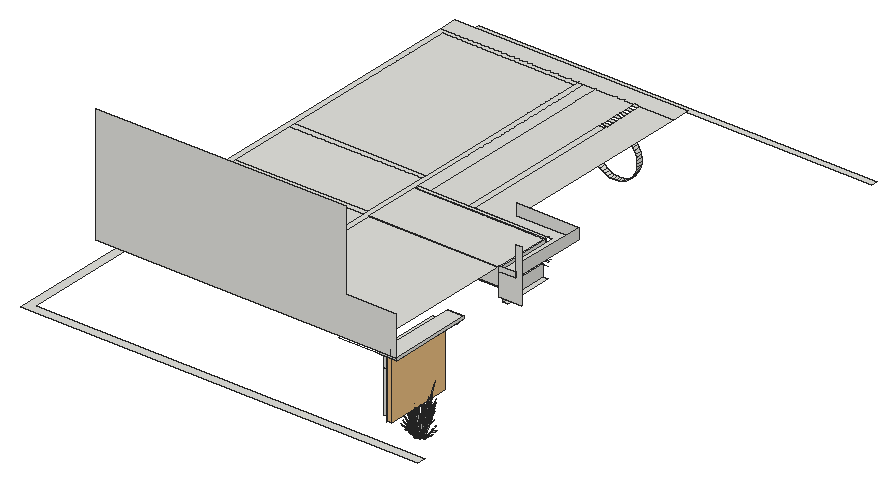
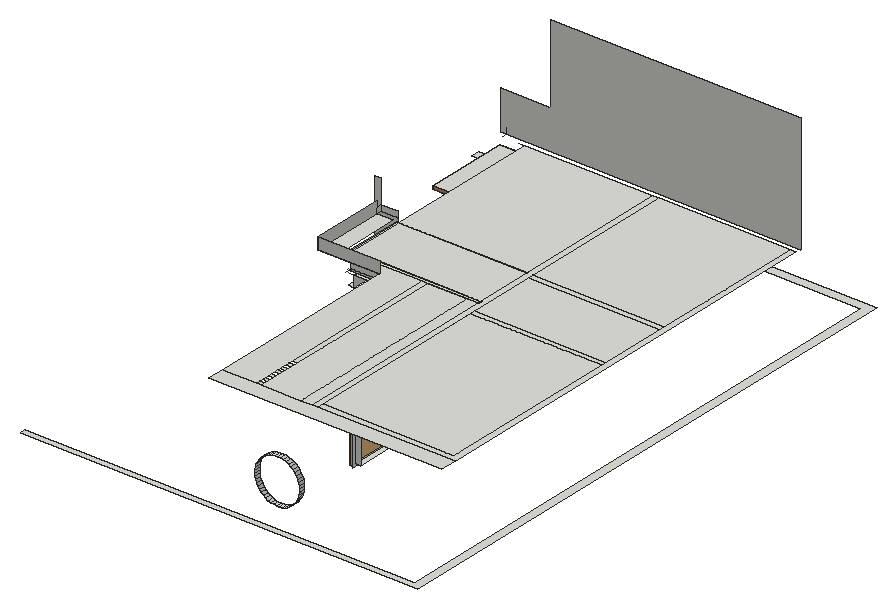
# SketchUp Ruby script. Lengths in inches.
U = 1.inch
M = Sketchup.active_model
def pt(a) = Geom::Point3d.new(a.map { |v| v * U })
def face(e, loops, mat)
  f = e.add_face(loops[0].map { |a| pt(a) })
  loops[1..].each { |l| e.add_face(l.map { |a| pt(a) }).erase! }
  f.material = f.back_material = mat if mat
  f
end
# faces: each face lists its corners as indices into pts; further lists are holes
def faces(e, pts, list, mat = nil) = list.each { |f| face(e, (f[0].is_a?(Array) ? f : [f]).map { |l| l.map { |i| pts[i] } }, mat) }
# xy, xz, yz: faces in a plane at the given z, y or x. An outline is a flat list of corners, or four numbers for a rectangle; further outlines are holes
def ring(l) = l.size == 4 ? [[l[0], l[1]], [l[2], l[1]], [l[2], l[3]], [l[0], l[3]]] : l.each_slice(2).to_a
def flat(e, list, mat, &to3) = list.each { |f| face(e, (f[0].is_a?(Array) ? f : [f]).map { |l| ring(l).map { |u, v| to3.(u, v) } }, mat) }
def xy(e, z, list, mat = nil) = flat(e, list, mat) { |x, y| [x, y, z] }
def xz(e, y, list, mat = nil) = flat(e, list, mat) { |x, z| [x, y, z] }
def yz(e, x, list, mat = nil) = flat(e, list, mat) { |y, z| [x, y, z] }
def lines(e, pts, list) = list.each { |a, b| e.add_line(pt(pts[a]), pt(pts[b])) }
# prism: a flat outline (further loops are holes) pulled along v
def prism(e, loops, v, mat = nil)
  f = face(e, loops, mat); d = Geom::Vector3d.new(v.map { |x| x * U })
  f.pushpull(f.normal.samedirection?(d) ? d.length : -d.length)
end
def box(e, o, s, mat = nil) = prism(e, [[o, [o[0] + s[0], o[1], o[2]], [o[0] + s[0], o[1] + s[1], o[2]], [o[0], o[1] + s[1], o[2]]]], [0, 0, s[2]], mat)
def at(x, y, z, deg = 0) = Geom::Transformation.translation(pt([x, y, z])) * Geom::Transformation.rotation(ORIGIN, Z_AXIS, deg.degrees)
def axes(o, x, y, z) = Geom::Transformation.new([*x, 0, *y, 0, *z, 0, *pt(o).to_a, 1])
def part(name) = M.definitions.add(name)
# library, detail: a bought-in or finely detailed component or shape, given as its bounding box
def library(name, o, s) = part(name).tap { |d| box(d.entities, o, s) }
def detail(e, o, s) = box(e.add_group.entities, o, s)
def put(e, d, t, mat = nil) = e.add_instance(d, t).tap { |i| i.material = mat if mat }
def group(e, t, mat = nil) = e.add_group.tap { |g| g.transformation = t; g.material = mat if mat }.entities
root = M.entities
M.materials.add("Brick_10_1K").color = [200, 136, 115]
M.materials.add("LightPink_Translucent").color = [144, 107, 117]
M.materials["LightPink_Translucent"].alpha = 0.75
c1 = part("blade")
p = [[2.15,0.21,22],[0,0.17,0],[0.09,0.45,0],[2.18,0.31,22],[2.29,0.31,22],[0.38,0.45,0],
  [2.48,0.24,33],[2.49,0.24,33],[2.48,0.22,33]]
faces(c1.entities,p,[[0,1,2,3],[4,5,2,3],[6,3,4,7],[8,0,3,6]])
c2 = part("seeds")
p = [[0.3,-0.1,1.38],[-0.01,-0.03,1.59],[-0.01,-0.03,0.03],[0.14,-0.07,-0.07],[0.29,-0.03,3],[0.15,0.01,3.11]]
faces(c2.entities,p,[[0,1,2,3],[1,0,4,5]],"LightPink_Translucent")
c3 = part("blade with seeds")
put(c3.entities,c1,at(0,0,0))
put(c3.entities,c2,axes([2.4,0.25,30.99],[1.5799,-0.05474,1.17369],[-0.12525,1.92788,0.29478],[-0.07173,-0.02425,1.56792]))
c4 = library("mesh-162",[-1607.75,-1245.64,-53.98],[1739.16,1702.88,120.91])
c5 = part("Group9\#1")
put(c5.entities,c4,at(0,0,0))
xy(root,39,[[192,384,198,450]])
xy(root,45,[[336,66,342,111],[336,111,342,132]])
xy(root,60,[[0,0,426,0,426,9,9,9,9,606.89,426,606.89,426,612.89,0,612.89]])
xy(root,84,[[336,225,342,279]])
xy(root,93,[[192,324,198,366],[192,384,198,450]])
xy(root,96,[[198,225,336,279]])
xy(root,111,[[342,54,360,63],[342,63,360,66],[336,66,360,132],[342,132,360,135],[342,135,360,138.72]])
xy(root,111,[[342,138.72,360,144]],"Brick_10_1K")
xy(root,114,[[342,54,360,144]])
xy(root,120,[[45,51,51,51,51,501,192,501,192,507,45,507],[51,51,192,219],[192,51,198,507],[198,51,336,219],[51,219,192,225],
  [198,219,336,281],[342,219,342,285,258,285,258,507,294,507,294,297,360,297,360,219],[336,219,338,281],[51,225,192,297],[198,281,336,285],
  [336,281,338,285],[198,285,210,507],[210,285,252,507],[252,285,258,459],[51,297,192,303],
  [51,303,192,501],[252,463,258,467],[252,471,258,475],[252,479,258,483],[252,487,258,491],
  [252,495,258,499],[252,503,258,507],[45,507,294,525]])
xz(root,45,[[45,120,366,120,366,162,312,162,312,246,45,246]])
xz(root,54,[[342,111,360,114]])
xz(root,66,[[336,45,342,90],[336,90,342,111]])
xz(root,132,[[336,45,342,111]])
xz(root,144,[[342,111,360,114]],"Brick_10_1K")
xz(root,213,[[342,96,366,96,366,151.99,360,151.99,360,120,342,120],[342,120,360,126]])
xz(root,219,[[198,102,336,120],[336,102,338,120]])
xz(root,281,[[198,100,338,102],[198,102,338,120]])
xz(root,297,[[294,120,360,132]])
xz(root,384,[[192,39,198,93]])
xz(root,450,[[192,39,198,93]])
yz(root,198,[[[381,36,453,96],[384,39,450,93]],[281,100,285,120]])
yz(root,336,[[225,84,279,96]])
yz(root,338,[[225,100,279,102],[279,100,281,102],[219,102,279,120]])
yz(root,342,[[63,42,135,42,135,111,132,111,132,45,66,45,66,111,63,111]])
yz(root,360,[[54,111,144,114],[213,120,219,126],[219,120,297,132]])
p = [[217.42,531,27.05],[214.41,531,27.11],[214.41,525,27.11],[217.42,525,27.05],[220.42,531,27.36],[220.42,525,27.36],
  [211.43,531,27.55],[211.43,525,27.55],[223.35,531,28.05],[223.35,525,28.05],[208.52,531,28.36],[208.52,525,28.36],
  [226.18,531,29.1],[226.18,525,29.1],[205.74,531,29.53],[205.74,525,29.53],[228.85,531,30.5],[228.85,525,30.5],
  [203.13,531,31.04],[203.13,525,31.04],[231.32,531,32.22],[231.32,525,32.22],[200.73,531,32.86],[200.73,525,32.86],
  [233.5625,531,34.24],[233.5625,525,34.24],[198.58,531,34.97],[198.58,525,34.97],[235.53,531,36.52],[235.53,525,36.52],
  [196.71,531,37.33],[196.71,525,37.33],[237.2,531,39.03],[237.2,525,39.03],[195.15,531,39.91],[195.15,525,39.91],
  [238.54,531,41.73],[238.54,525,41.73],[193.92,531,42.66],[193.92,525,42.66],[239.53,531,44.58],[239.53,525,44.58],
  [193.05,531,45.54],[193.05,525,45.54],[240.16,531,47.52],[240.16,525,47.52],[192.55,531,48.52],[192.55,525,48.52],
  [240.41,531,50.53],[240.41,525,50.53],[192.42,531,51.53],[192.42,525,51.53],[240.28,531,53.54],[240.28,525,53.54],
  [192.67,531,54.53],[192.67,525,54.53],[239.78,531,56.51],[239.78,525,56.51],[193.3,531,57.48],[193.3,525,57.48],
  [238.91,531,59.4],[238.91,525,59.4],[194.29,531,60.33],[194.29,525,60.33],[237.68,531,62.15],[237.68,525,62.15],
  [195.63,531,63.03],[195.63,525,63.03],[236.12,531,64.73],[236.12,525,64.73],[197.3,531,65.54],[197.3,525,65.54],
  [234.25,531,67.09],[234.25,525,67.09],[199.27,531,67.82],[199.27,525,67.82],[232.09,531,69.2],[232.09,525,69.2],
  [201.5,531,69.83],[201.5,525,69.83],[229.69,531,71.02],[229.69,525,71.02],[203.98,531,71.55],[203.98,525,71.55],
  [227.08,531,72.53],[227.08,525,72.53],[206.65,531,72.95],[206.65,525,72.95],[224.3,531,73.69],[224.3,525,73.69],
  [209.48,531,74],[209.48,525,74],[221.4,531,74.5],[221.4,525,74.5],[212.41,531,74.69],[212.41,525,74.69],
  [218.42,531,74.94],[218.42,525,74.94],[215.41,531,75.01],[215.41,525,75.01],[340,283,100],[340,285,100],
  [342,54,111],[297.24,54,111],[338,281,100],[342,281,100],[338,225,100],[342,225,100],
  [338,279,100],[342,279,100],[336,225,96],[342,225,96],[336,279,96],[342,279,96],
  [360,45,120],[360,45,126],[360,51,120],[336,51,120],[342,51,120]]
faces(root,p,[[0,1,2,3],[4,0,3,5],[1,6,7,2],[8,4,5,9],[6,10,11,7],[12,8,9,13],[10,14,15,11],[16,12,13,17],
  [14,18,19,15],[20,16,17,21],[18,22,23,19],[24,20,21,25],[22,26,27,23],[28,24,25,29],[26,30,31,27],[32,28,29,33],
  [30,34,35,31],[36,32,33,37],[34,38,39,35],[40,36,37,41],[38,42,43,39],[44,40,41,45],[42,46,47,43],[48,44,45,49],
  [46,50,51,47],[52,48,49,53],[50,54,55,51],[56,52,53,57],[54,58,59,55],[60,56,57,61],[58,62,63,59],[64,60,61,65],
  [62,66,67,63],[68,64,65,69],[66,70,71,67],[72,68,69,73],[70,74,75,71],[76,72,73,77],[74,78,79,75],[80,76,77,81],
  [78,82,83,79],[84,80,81,85],[82,86,87,83],[88,84,85,89],[86,90,91,87],[92,88,89,93],[90,94,95,91],[96,92,93,97],
  [94,98,99,95],[98,96,97,99]])
lines(root,p,[[100,101],[102,103],[104,105],[106,107],[108,109],[110,111],[112,113],[114,115],[116,114],[117,118]])
put(root,c3,axes([347.28,106.03,11.03],[0.0479,-0.66354,-0.1216],[0.90696,0.01814,-0.67495],[0.3493,0.04609,1.02557]))
put(root,c3,axes([340.5,103.49,11.03],[0.45012,0.59081,-0.1216],[-0.79888,0.29033,-0.67495],[-0.33665,0.07795,1.02557]))
put(root,c3,axes([347.19,102.2,11.03],[-0.98321,-0.03233,-0.1216],[0.02687,-0.61208,-0.67495],[0.0683,-0.23574,1.02557]))
put(root,c3,axes([348.29,104.8,11.03],[-0.45012,-0.59081,-0.1216],[0.79888,-0.29033,-0.67495],[0.33665,-0.07795,1.02557]))
put(root,c3,axes([343.42,106.78,11.03],[0.87543,-0.30377,-0.1216],[0.4302,0.53915,-0.67495],[0.1155,0.2272,1.02557]))
put(root,c3,axes([341.51,102.26,11.03],[-0.0479,0.66354,-0.1216],[-0.90696,-0.01814,-0.67495],[-0.3493,-0.04609,1.02557]))
put(root,c3,axes([345.5,106.75,11.03],[0.53309,-0.55848,-0.1216],[0.77201,0.32175,-0.67495],[0.26836,0.15779,1.02557]))
put(root,c3,axes([340.53,104.89,11.03],[0.82753,0.35977,-0.1216],[-0.47675,0.52101,-0.67495],[-0.2338,0.18111,1.02557]))
put(root,c3,axes([345.37,101.51,11.03],[-0.87543,0.30377,-0.1216],[-0.4302,-0.53915,-0.67495],[-0.1155,-0.2272,1.02557]))
put(root,c3,axes([348.26,103.4,11.03],[-0.82753,-0.35977,-0.1216],[0.47675,-0.52101,-0.67495],[0.2338,-0.18111,1.02557]))
put(root,c3,axes([346.1,103.46,10.47],[-0.77304,-0.33901,1.38283],[0.81626,-0.52782,0.59665],[0.24941,0.31809,1.33663]))
put(root,c3,axes([339.56,104.08,10.72],[-0.14609,0.08471,1.74944],[0.01243,0.61893,-0.27667],[-0.33486,0.08049,0.14031]))
put(root,c3,axes([350.74,103.88,10.72],[0.12414,-0.09938,1.74944],[-0.15889,-0.60963,-0.27667],[0.31148,-0.11559,0.14031]))
put(root,c3,axes([348.07,105.63,10.72],[0.19191,-0.01103,1.74944],[0.52639,-0.5069,-0.27667],[0.34136,0.06691,0.14031]))
put(root,c3,axes([348.09,101.22,10.72],[-0.00864,-0.12985,1.74944],[-0.72937,-0.3753,-0.27667],[0.11277,-0.2275,0.14031]))
put(root,c3,axes([339.58,106.39,10.72],[-0.02224,0.12912,1.74944],[0.63107,0.44917,-0.27667],[-0.16521,0.21241,0.14031]))
put(root,c3,axes([343.21,107.98,10.72],[0.1134,0.10507,1.74944],[0.91515,0.04128,-0.27667],[0.09203,0.23172,0.14031]))
put(root,c3,axes([343.98,100.1,10.72],[-0.13683,-0.09148,1.74944],[-0.91315,0.058,-0.27667],[-0.14574,-0.2188,0.14031]))
put(root,c3,axes([340.99,101.11,10.72],[-0.19249,-0.00461,1.74944],[-0.61281,0.46055,-0.27667],[-0.32697,-0.0941,0.14031]))
put(root,c3,axes([340.25,101.5,10.71],[0.06632,0.06511,1.77383],[-0.31973,0.58531,-0.16761],[-0.32381,0.00424,0.31391]))
put(root,c3,axes([343.05,99.8,10.71],[-0.01669,0.07821,1.77383],[-0.82314,0.28383,-0.16761],[-0.24223,-0.14508,0.31391]))
put(root,c3,axes([344.8,107.22,10.71],[0.00265,-0.07899,1.77383],[0.76665,-0.34851,-0.16761],[0.2663,0.12439,0.31391]))
put(root,c3,axes([337.93,104.7,10.71],[0.11417,0.0175,1.77383],[0.35319,0.57649,-0.16761],[-0.23371,0.15131,0.31391]))
put(root,c3,axes([350.3,103.24,10.71],[-0.11685,-0.00496,1.77383],[-0.48522,-0.53096,-0.16761],[0.19486,-0.17458,0.31391]))
put(root,c3,axes([350.09,106.56,10.71],[-0.08089,-0.05712,1.77383],[0.17695,-0.61228,-0.16761],[0.31864,-0.03912,0.31391]))
put(root,c3,axes([339.51,107.71,10.71],[0.10149,-0.03939,1.77383],[0.83886,0.26202,-0.16761],[-0.01971,0.21816,0.31391]))
put(root,c3,axes([347.89,100.76,10.71],[-0.09085,0.04984,1.77383],[-0.89014,-0.16814,-0.16761],[-0.03222,-0.21748,0.31391]))
put(root,c3,axes([341.6,106.09,11.4],[0.98321,0.03233,-0.13498],[-0.02687,0.61208,-0.74919],[-0.0683,0.23574,1.13838]))
put(root,c3,axes([343.28,101.29,11.43],[-0.59706,0.6255,-0.13619],[-0.86465,-0.36036,-0.75594],[-0.30056,-0.17672,1.14864]))
put(root,c3,axes([343.09,101.33,10.73],[0.4066,-0.41448,0.0643],[0.57901,0.24131,0.50621],[-0.18719,-0.13288,0.77189]))
put(root,c3,axes([343.4375,107.02,10.73],[-0.6592,0.22175,0.0643],[-0.32265,-0.40436,0.50621],[0.06366,0.17825,0.77189]))
put(root,c3,axes([348.5625,103.27,10.73],[0.61415,0.2744,0.0643],[-0.35756,0.39076,0.50621],[0.1969,-0.12633,0.77189]))
put(root,c3,axes([348.66,104.79,10.73],[0.32857,0.44488,0.0643],[-0.59916,0.21775,0.50621],[0.26412,-0.04296,0.77189]))
put(root,c3,axes([341.19,102.15,10.73],[0.04505,-0.49615,0.0643],[0.68022,0.0136,0.50621],[-0.26056,-0.05192,0.77189]))
put(root,c3,axes([347.36,101.98,10.73],[0.73517,0.0304,0.0643],[-0.02016,0.45906,0.50621],[0.07693,-0.17585,0.77189]))
put(root,c3,axes([347.61,106.14,10.73],[-0.04505,0.49615,0.0643],[-0.68022,-0.0136,0.50621],[0.26056,0.05192,0.77189]))
put(root,c3,axes([340.23,105.02,10.73],[-0.61415,-0.2744,0.0643],[0.35756,-0.39076,0.50621],[-0.1969,0.12633,0.77189]))
put(root,c3,axes([345.35,101.27,10.73],[0.6592,-0.22175,0.0643],[0.32265,0.40436,0.50621],[-0.06366,-0.17825,0.77189]))
put(root,c3,axes([340.14,103.5,10.73],[-0.32857,-0.44488,0.0643],[0.59916,-0.21775,0.50621],[-0.26412,0.04296,0.77189]))
put(root,c3,axes([345.7,106.96,10.73],[-0.4066,0.41448,0.0643],[-0.57901,-0.24131,0.50621],[0.18719,0.13288,0.77189]))
put(root,c3,axes([341.4375,106.3125,10.73],[-0.73517,-0.0304,0.0643],[0.02016,-0.45906,0.50621],[-0.07693,0.17585,0.77189]))
put(root,c3,axes([345.12,101.3125,10.73],[0.88151,0.17057,0.48003],[-0.30143,0.56078,0.3958],[-0.05297,-0.22053,0.9933]))
put(root,c3,axes([347.67,105.98,10.73],[-0.65964,0.42992,0.48003],[-0.5689,-0.45657,0.3958],[0.30948,0.0793,0.9933]))
put(root,c3,axes([348.59,104.63,10.73],[-0.25275,0.59491,0.48003],[-0.83094,-0.20343,0.3958],[0.32677,-0.03575,0.9933]))
put(root,c3,axes([340.4,105.14,10.73],[-0.22187,-0.60049,0.48003],[0.87033,-0.10422,0.3958],[-0.25651,0.14123,0.9933]))
put(root,c3,axes([341.67,106.35,10.73],[-0.63704,-0.44518,0.48003],[0.67652,-0.38394,0.3958],[-0.11751,0.20886,0.9933]))
put(root,c3,axes([347.12,101.9375,10.73],[0.63704,0.44518,0.48003],[-0.67652,0.38394,0.3958],[0.11751,-0.20886,0.9933]))
put(root,c3,axes([340.2,103.66,10.73],[0.25275,-0.59491,0.48003],[0.83094,0.20343,0.3958],[-0.32677,0.03575,0.9933]))
put(root,c3,axes([348.39,103.15,10.73],[0.22187,0.60049,0.48003],[-0.87033,0.10422,0.3958],[0.25651,-0.14123,0.9933]))
put(root,c3,axes([345.87,106.84,10.73],[-0.88979,0.14973,0.48003],[-0.15442,-0.58737,0.3958],[0.20926,0.17311,0.9933]))
put(root,c3,axes([343.68,106.57,11.05],[0.2697,-0.50175,0.35414],[0.78684,0.14635,-0.4572],[0.07215,0.20201,0.87481]))
put(root,c3,axes([345.11,101.72,11.05],[-0.2697,0.50175,0.35414],[-0.78684,-0.14635,-0.4572],[-0.07215,-0.20201,0.87481]))
put(root,c3,axes([347.14,105.77,11.05],[-0.50902,-0.40851,0.35414],[0.58122,-0.38671,-0.4572],[0.29531,0.05884,0.87481]))
put(root,c3,axes([347.98,104.625,11.05],[-0.74348,-0.18202,0.35414],[0.21685,-0.53102,-0.4572],[0.29933,-0.04869,0.87481]))
put(root,c3,axes([341.65,102.52,11.05],[0.50902,0.40851,0.35414],[-0.58122,0.38671,-0.4572],[-0.29531,-0.05884,0.87481]))
put(root,c3,axes([341.98,106,11.05],[0.60531,-0.34352,0.35414],[0.573,0.39225,-0.4572],[-0.08718,0.19929,0.87481]))
put(root,c3,axes([340.93,104.9375,11.05],[0.77872,-0.09325,0.35414],[0.20563,0.53305,-0.4572],[-0.22316,0.14318,0.87481]))
put(root,c3,axes([345.57,106.48,11.05],[-0.13817,-0.52554,0.35414],[0.78985,-0.13877,-0.4572],[0.21215,0.1506,0.87481]))
put(root,c3,axes([347.86,103.35,11.05],[-0.77872,0.09325,0.35414],[-0.20563,-0.53305,-0.4572],[0.22316,-0.14318,0.87481]))
put(root,c3,axes([340.81,103.66,11.05],[0.74348,0.18202,0.35414],[-0.21685,0.53102,-0.4572],[-0.29933,0.04869,0.87481]))
put(root,c3,axes([346.81,102.29,11.05],[-0.60531,0.34352,0.35414],[-0.573,-0.39225,-0.4572],[0.08718,-0.19929,0.87481]))
put(root,c3,axes([343.22,101.81,11.05],[0.13817,0.52554,0.35414],[-0.78985,0.13877,-0.4572],[-0.21215,-0.1506,0.87481]))
put(root,c3,axes([343.67,106.98,11.0625],[-0.88151,-0.17057,0.53283],[0.30143,-0.56078,0.43934],[0.05297,0.22053,1.10256]))
put(root,c3,axes([340.85,102.15,11.09],[0.7388,-0.48151,0.53763],[0.63717,0.51135,0.4433],[-0.34662,-0.08882,1.11249]))
put(root,c3,axes([342.87,101.19,11.09],[0.99656,-0.1677,0.53763],[0.17295,0.65785,0.4433],[-0.23438,-0.19388,1.11249]))
put(root,c3,axes([344.74,108.36,11.65],[0.61821,-0.37431,-0.06488],[0.56645,0.40995,-0.29416],[0.03988,0.11616,0.97024]))
put(root,c3,axes([339.17,106.45,11.65],[0.78943,0.17416,-0.06488],[-0.24284,0.53604,-0.29416],[-0.12912,0.08139,0.97024]))
put(root,c5,axes([200.27,433.3,91.55],[0,0,0.03386],[0,0.04198,0],[-0.03386,0,0]))
put(root,c5,axes([344.63,115.47,105.83],[0,0,0.03937],[0,0.04213,0],[-0.03937,0,0]))
